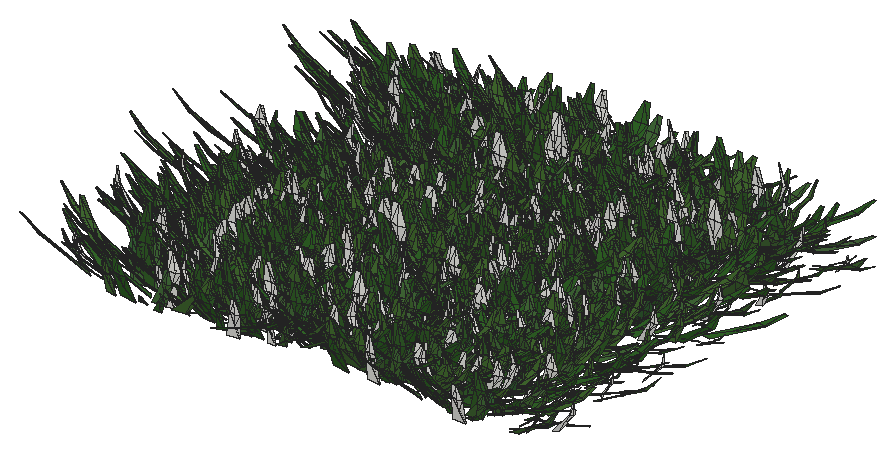
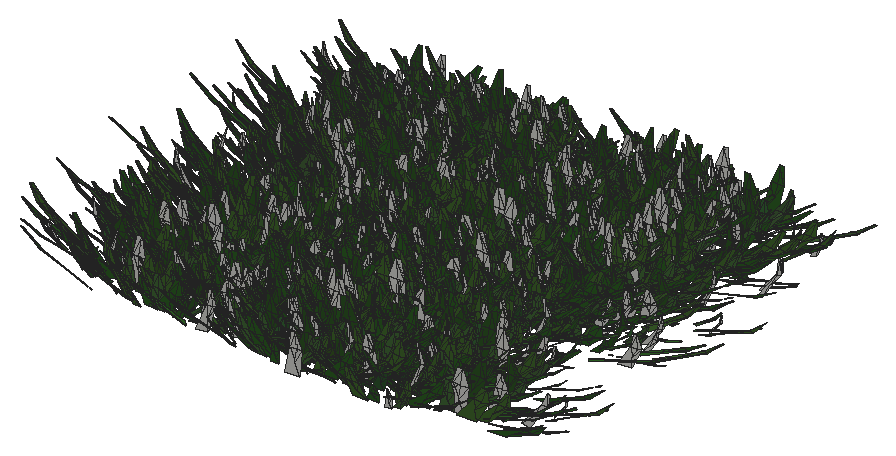
# SketchUp Ruby script. Lengths in inches.
U = 1.inch
M = Sketchup.active_model
def pt(a) = Geom::Point3d.new(a.map { |v| v * U })
def face(e, loops, mat)
  f = e.add_face(loops[0].map { |a| pt(a) })
  loops[1..].each { |l| e.add_face(l.map { |a| pt(a) }).erase! }
  f.material = f.back_material = mat if mat
  f
end
# faces: each face lists its corners as indices into pts; further lists are holes
def faces(e, pts, list, mat = nil) = list.each { |f| face(e, (f[0].is_a?(Array) ? f : [f]).map { |l| l.map { |i| pts[i] } }, mat) }
# xy, xz, yz: faces in a plane at the given z, y or x. An outline is a flat list of corners, or four numbers for a rectangle; further outlines are holes
def ring(l) = l.size == 4 ? [[l[0], l[1]], [l[2], l[1]], [l[2], l[3]], [l[0], l[3]]] : l.each_slice(2).to_a
def flat(e, list, mat, &to3) = list.each { |f| face(e, (f[0].is_a?(Array) ? f : [f]).map { |l| ring(l).map { |u, v| to3.(u, v) } }, mat) }
def xy(e, z, list, mat = nil) = flat(e, list, mat) { |x, y| [x, y, z] }
def xz(e, y, list, mat = nil) = flat(e, list, mat) { |x, z| [x, y, z] }
def yz(e, x, list, mat = nil) = flat(e, list, mat) { |y, z| [x, y, z] }
def lines(e, pts, list) = list.each { |a, b| e.add_line(pt(pts[a]), pt(pts[b])) }
# prism: a flat outline (further loops are holes) pulled along v
def prism(e, loops, v, mat = nil)
  f = face(e, loops, mat); d = Geom::Vector3d.new(v.map { |x| x * U })
  f.pushpull(f.normal.samedirection?(d) ? d.length : -d.length)
end
def box(e, o, s, mat = nil) = prism(e, [[o, [o[0] + s[0], o[1], o[2]], [o[0] + s[0], o[1] + s[1], o[2]], [o[0], o[1] + s[1], o[2]]]], [0, 0, s[2]], mat)
def at(x, y, z, deg = 0) = Geom::Transformation.translation(pt([x, y, z])) * Geom::Transformation.rotation(ORIGIN, Z_AXIS, deg.degrees)
def axes(o, x, y, z) = Geom::Transformation.new([*x, 0, *y, 0, *z, 0, *pt(o).to_a, 1])
def part(name) = M.definitions.add(name)
# library, detail: a bought-in or finely detailed component or shape, given as its bounding box
def library(name, o, s) = part(name).tap { |d| box(d.entities, o, s) }
def detail(e, o, s) = box(e.add_group.entities, o, s)
def put(e, d, t, mat = nil) = e.add_instance(d, t).tap { |i| i.material = mat if mat }
def group(e, t, mat = nil) = e.add_group.tap { |g| g.transformation = t; g.material = mat if mat }.entities
root = M.entities
M.materials.add("Material10").color = [48, 100, 38]
M.materials.add("Material3").color = [68, 110, 58]
M.materials.add("Material4").color = [48, 90, 38]
M.materials.add("Material5").color = [68, 110, 48]
M.materials.add("Material6").color = [48, 90, 48]
M.materials.add("Material7").color = [58, 110, 58]
M.materials.add("Material8").color = [58, 90, 38]
M.materials.add("Material9").color = [68, 100, 58]
c1 = part("grass00")
p = [[-0.6875,0.15,0],[-0.56,0.08,5.52],[-0.04,0.03,2.76],[0.48,-0.02,0],[0.35,-0.02,5.52],[-0.1,-0.14,5.52],
  [-0.12,0.65,8.37],[-0.42,0.65,8.37]]
faces(c1.entities,p,[[0,1,2,3],[3,2,4],[1,5,2],[5,4,2],[1,6,5],[4,5,6],[7,6,1]])
c2 = part("Group16\#1")
put(c2.entities,c1,axes([1.44,-0.61,-0.01],[0.05352,0.12609,0],[-0.10704,0.04543,0.07239],[0.06664,-0.02828,0.11628]),"Material6")
put(c2.entities,c1,axes([0.76,-0.15,-0.01],[0.04676,0.24062,0],[-0.23162,0.04501,0.06642],[0.0652,-0.01267,0.23595]),"Material3")
put(c2.entities,c1,axes([0.79,0.01,-0.01],[-0.00606,0.34651,0],[-0.34381,-0.00602,0.0432],[0.04319,0.00076,0.34386]))
put(c2.entities,c1,axes([1,0.23,-0.01],[-0.07192,0.31144,0],[-0.28722,-0.06632,0.1236],[0.12043,0.02781,0.29478]),"Material5")
put(c2.entities,c1,axes([1.66,0.77,-0.01],[-0.13828,0.29651,0],[-0.21551,-0.1005,0.22471],[0.20365,0.09498,0.23779]),"Material10")
put(c2.entities,c1,axes([0.6875,0.52,-0.01],[-0.18126,0.24051,0],[-0.22746,-0.17142,0.09788],[0.07817,0.05891,0.28481]),"Material5")
put(c2.entities,c1,axes([0.68,0.78,-0.01],[-0.215,0.18688,0],[-0.12385,-0.14248,0.21334],[0.13995,0.16101,0.18878]),"Material3")
put(c2.entities,c1,axes([0.56,1,-0.01],[-0.13756,0.07624,0],[-0.06159,-0.11112,0.0927],[0.04494,0.08108,0.12705]),"Material5")
put(c2.entities,c1,axes([0.2,0.64,-0.01],[-0.23729,0.07254,0],[-0.05711,-0.18681,0.153],[0.04473,0.14632,0.19535]),"Material10")
put(c2.entities,c1,axes([0.0625,0.72,-0.01],[-0.28874,0.02525,0],[-0.02179,-0.24916,0.14647],[0.01276,0.14591,0.25012]),"Material3")
put(c2.entities,c1,axes([-0.08,0.62,-0.01],[-0.34089,-0.04187,0],[0.03255,-0.26504,0.216],[-0.02633,0.21439,0.26703]),"Material10")
put(c2.entities,c1,axes([-0.34,0.98,-0.01],[-0.14314,-0.0493,0],[0.04397,-0.12769,0.06843],[-0.02228,0.0647,0.13505]),"Material10")
put(c2.entities,c1,axes([-0.87,1.45,-0.01],[-0.23488,-0.14114,0],[0.13761,-0.22901,0.06087],[-0.03135,0.05217,0.26717]))
put(c2.entities,c1,axes([-0.72,0.77,-0.01],[-0.14208,-0.13251,0],[0.07209,-0.0773,0.16301],[-0.11118,0.11922,0.1057]),"Material10")
put(c2.entities,c1,axes([-0.62,0.43,-0.01],[-0.14845,-0.21203,0],[0.18654,-0.13061,0.12304],[-0.10079,0.07057,0.22772]),"Material3")
put(c2.entities,c1,axes([-0.68,0.29,-0.01],[-0.13639,-0.32136,0],[0.31723,-0.13464,0.05579],[-0.05136,0.0218,0.34462]),"Material4")
put(c2.entities,c1,axes([-0.64,0.125,-0.01],[-0.0458,-0.23569,0],[0.22124,-0.043,0.08276],[-0.08124,0.01579,0.22538]),"Material7")
put(c2.entities,c1,axes([-1.6,-0.03,-0.01],[0.00576,-0.32897,0],[0.27526,0.00482,0.18018],[-0.18015,-0.00315,0.2753]),"Material5")
put(c2.entities,c1,axes([-1.36,-0.31,-0.01],[0.05718,-0.24765,0],[0.18172,0.04196,0.17267],[-0.16825,-0.03885,0.1865]),"Material10")
put(c2.entities,c1,axes([-1.54,-0.72,-0.01],[0.06537,-0.14017,0],[0.13555,0.06321,0.03939],[-0.0357,-0.01665,0.14956]))
put(c2.entities,c1,axes([-1.19,-0.9,-0.01],[0.09597,-0.12735,0],[0.11214,0.08451,0.07557],[-0.06035,-0.04548,0.14042]),"Material9")
put(c2.entities,c1,axes([-0.47,-0.54,-0.01],[0.11588,-0.10072,0],[0.0618,0.0711,0.12124],[-0.07953,-0.0915,0.0942]))
put(c2.entities,c1,axes([-0.47,-0.84,-0.01],[0.11927,-0.0661,0],[0.06603,0.11913,0.00646],[-0.00313,-0.00565,0.13621]),"Material5")
put(c2.entities,c1,axes([-0.38,-1.24,-0.01],[0.28037,-0.08571,0],[0.0618,0.20215,0.20315],[-0.05939,-0.19428,0.21139]),"Material9")
put(c2.entities,c1,axes([-0.06,-0.66,-0.01],[0.22719,-0.01987,0],[0.01247,0.14255,0.17758],[-0.01547,-0.17691,0.1431]),"Material8")
put(c2.entities,c1,axes([0.11,-0.89,-0.01],[0.14882,0.01828,0],[-0.01058,0.08611,0.12229],[0.01491,-0.12138,0.08676]),"Material6")
put(c2.entities,c1,axes([0.25,-0.72,-0.01],[0.20481,0.07053,0],[-0.06206,0.18022,0.10291],[0.03351,-0.0973,0.1906]),"Material6")
put(c2.entities,c1,axes([0.85,-1.42,-0.01],[0.16481,0.09904,0],[-0.09472,0.15762,0.05616],[0.02893,-0.04814,0.18389]),"Material5")
put(c2.entities,c1,axes([1.01,-1.09,-0.01],[0.21858,0.20385,0],[-0.17495,0.1876,0.15339],[0.10462,-0.11218,0.25652]),"Material10")
put(c2.entities,c1,axes([1.01,-0.71,-0.01],[0.08733,0.12473,0],[-0.06445,0.04512,0.13037],[0.1068,-0.07477,0.07867]),"Material6")
c3 = part("Group15\#1")
put(c3.entities,c2,at(0,0,0))
c4 = part("3darcstudiotree_grass00\#1")
put(c4.entities,c3,at(0,0,0))
put(root,c4,axes([226.21,4.08,7.6],[3.20529,-0.95815,0],[3.41522,0.71406,-0.02296],[0.11616,0.02429,1.8355]))
put(root,c4,axes([225.98,41.5625,7.6],[-1.06603,0.92748,0],[-4.93521,-0.35453,-0.06106],[-0.26936,-0.01935,1.47293]))
put(root,c4,axes([225.79,20.19,7.6],[5.08676,-0.19422,0],[0.58185,0.95246,-0.02943],[0.02798,0.0458,1.51666]))
put(root,c4,axes([227.38,18.53,7.6],[-0.19939,-1.04542,0],[4.4829,-0.05344,-0.05646],[0.31576,-0.00376,1.57058]))
put(root,c4,axes([225.93,11.33,7.6],[2.71383,0.81638,0],[-3.43896,0.71449,-0.05468],[-0.2392,0.0497,1.58958]))
put(root,c4,axes([225.9,26.8,7.6],[4.84098,0.43489,0],[-1.61189,1.12141,-0.03831],[-0.06664,0.04636,1.53223]))
put(root,c4,axes([226.47,38.5,7.6],[4.94595,-0.11829,0],[0.37031,0.96768,-0.00501],[0.00319,0.00833,1.62495]))
put(root,c4,axes([226.14,12.84,7.6],[2.55592,1.10469,0],[-4.04438,0.58485,-0.02506],[-0.13578,0.01964,1.82822]))
put(root,c4,axes([226.78,7.125,7.6],[4.08301,-0.07651,0],[0.38191,1.27383,-0.00347],[0.00157,0.00523,1.92949]))
put(root,c4,axes([227.87,35.8,7.6],[-2.35704,0.79519,0],[-3.72282,-0.68968,-0.05517],[-0.2648,-0.04906,1.72999]))
put(root,c4,axes([227.11,17.55,7.6],[2.61917,0.95948,0],[-3.03892,0.51848,-0.01403],[-0.09978,0.01702,1.97952]))
put(root,c4,axes([227.21,23.57,7.6],[3.34714,0.66833,0],[-2.79001,0.87331,-0.04015],[-0.12528,0.03922,1.39698]))
put(root,c4,axes([227.82,14.5625,7.6],[0.48467,1.00987,0],[-3.72895,0.11185,-0.01784],[-0.13598,0.00408,1.80168]))
put(root,c4,axes([229.61,33.6875,7.6],[-1.59666,-0.99905,0],[3.40836,-0.34045,-0.01431],[0.10062,-0.01005,1.73701]))
put(root,c4,axes([229.78,5.64,7.6],[-3.03643,0.87412,0],[-2.8621,-0.62138,-0.01448],[-0.06458,-0.01402,1.39954]))
put(root,c4,axes([230.84,6.7,7.6],[-4.02149,-0.43578,0],[1.45299,-0.83803,-0.04544],[0.11799,-0.06805,1.4908]))
put(root,c4,axes([231.12,29.33,7.6],[-4.89707,0.28407,0],[-0.88262,-0.95096,-0.03599],[-0.04789,-0.0516,1.43677]))
put(root,c4,axes([230.44,14.26,7.6],[-3.37258,0.90608,0],[-3.64602,-0.8482,-0.01383],[-0.04832,-0.01124,1.48532]))
put(root,c4,axes([229.94,22.19,7.6],[4.28972,0.40809,0],[-1.53876,1.01093,-0.01203],[-0.02546,0.01673,1.60927]))
put(root,c4,axes([231.98,18.82,7.6],[-1.14965,-0.87516,0],[3.85465,-0.31648,-0.02104],[0.11481,-0.00943,1.45661]))
put(root,c4,axes([231.18,16.43,7.6],[3.45148,-0.64536,0],[2.96079,0.98967,-0.02614],[0.07518,0.02513,1.48366]))
put(root,c4,axes([232.02,20.76,7.6],[-4.9983,0.12378,0],[-0.36429,-0.91937,-0.0174],[-0.01281,-0.03234,1.72585]))
put(root,c4,axes([232.56,38.6,7.6],[-3.38152,-0.37053,0],[1.95757,-1.11657,-0.00176],[0.00453,-0.00258,1.95594]))
put(root,c4,axes([231.52,11.12,7.6],[-2.34957,0.94392,0],[-4.17021,-0.64877,-0.04897],[-0.26523,-0.04126,1.9584]))
put(root,c4,axes([230.93,8.84,7.6],[3.32402,0.3596,0],[-1.44399,0.83424,-0.02703],[-0.09074,0.05242,1.9211]))
put(root,c4,axes([232.95,26.33,7.6],[-3.05623,-0.47682,0],[2.41216,-0.96631,-0.00523],[0.01811,-0.00725,1.86317]))
put(root,c4,axes([233.09,28.7,7.6],[-3.75382,-0.50938,0],[2.09214,-0.9636,-0.04387],[0.13012,-0.05993,1.70431]))
put(root,c4,axes([232.33,9.76,7.6],[-3.73599,0.53776,0],[-2.5701,-1.11595,-0.0199],[-0.05158,-0.02239,1.67187]))
put(root,c4,axes([231.25,25.49,7.6],[1.67846,0.81167,0],[-4.27264,0.55222,-0.03477],[-0.1745,0.02255,1.69826]))
put(root,c4,axes([232.66,17.13,7.6],[-3.09646,0.77516,0],[-3.18498,-0.79517,-0.05526],[-0.23608,-0.05894,1.69871]))
put(root,c4,axes([232.67,12.55,7.6],[2.62671,-0.96021,0],[3.1714,0.54222,-0.02882],[0.14083,0.02408,1.42183]))
put(root,c4,axes([233.14,43.38,7.6],[0.41254,-1.11538,0],[3.92373,0.0907,-0.04487],[0.25663,0.00593,1.41449]))
put(root,c4,axes([233.58,42.34,7.6],[-4.83141,-0.06367,0],[0.25709,-1.21932,-0.0488],[0.01394,-0.06614,1.65721]))
put(root,c4,axes([233.43,4.38,7.6],[-3.80323,0.13534,0],[-0.55678,-0.97788,-0.03826],[-0.03613,-0.06345,1.65468]))
put(root,c4,axes([234.05,39.82,7.6],[-4.67907,-0.20575,0],[0.86048,-1.22305,-0.04722],[0.03699,-0.05257,1.40384]))
put(root,c4,axes([232.57,36.71,7.6],[-1.05875,1.15742,0],[-4.29725,-0.24568,-0.0233],[-0.13048,-0.00746,1.58282]))
put(root,c4,axes([232.625,23.74,7.6],[4.14871,0.66652,0],[-2.80307,1.09047,-0.03131],[-0.07779,0.03026,1.48921]))
put(root,c4,axes([232.9,32.76,7.6],[2.97201,1.00736,0],[-3.97981,0.73385,-0.05484],[-0.18767,0.03461,1.31443]))
put(root,c4,axes([233.51,31.37,7.6],[3.73635,0.02915,0],[-0.121,0.9694,-0.01718],[-0.00416,0.0333,1.88076]))
put(root,c4,axes([235.78,16.42,7.6],[-3.38708,-0.63927,0],[2.81669,-0.93274,-0.01411],[0.04933,-0.01634,1.69584]))
put(root,c4,axes([233.76,35.375,7.6],[0.16986,1.07544,0],[-5.18803,0.05121,-0.04149],[-0.19714,0.00195,1.54325]))
put(root,c4,axes([235.98,29.46,7.6],[0.73918,-1.25402,0],[4.5803,0.16874,-0.00777],[0.03593,0.00132,1.3523]))
put(root,c4,axes([236.16,26.67,7.6],[-0.83171,-0.90909,0],[4.59832,-0.26293,-0.04627],[0.28513,-0.0163,1.86363]))
put(root,c4,axes([236.2,17.17,7.6],[-4.52783,0.09424,0],[-0.31079,-0.93327,-0.02559],[-0.01771,-0.05318,1.95328]))
put(root,c4,axes([237.05,25.02,7.6],[1.09611,-0.92163,0],[4.84666,0.36027,-0.06029],[0.32691,0.0243,1.78762]))
put(root,c4,axes([236.72,39.72,7.6],[2.30561,-0.85947,0],[4.07199,0.68272,-0.05795],[0.30529,0.05118,1.94389]))
put(root,c4,axes([236.01,8.4,7.6],[4.15645,0.11327,0],[-0.40548,0.92998,-0.03498],[-0.02406,0.05518,1.48455]))
put(root,c4,axes([236.93,21.94,7.6],[-3.28835,0.69112,0],[-2.3207,-0.69011,-0.00081],[-0.00409,-0.00122,1.76997]))
put(root,c4,axes([238.16,34.58,7.6],[-0.05217,-0.99103,0],[4.9332,-0.01623,-0.00745],[0.04692,-0.00015,1.94284]))
put(root,c4,axes([236.73,5.44,7.6],[0.29849,1.1081,0],[-3.91006,0.06583,-0.04154],[-0.31526,0.00531,1.86323]))
put(root,c4,axes([238.3125,31.26,7.6],[-4.94093,-0.24625,0],[0.95755,-1.20083,-0.01918],[0.02332,-0.02924,1.90358]))
put(root,c4,axes([236.96,36.09,7.6],[3.27459,-0.53526,0],[2.01,0.76855,-0.045],[0.14728,0.05631,1.37282]))
put(root,c4,axes([238.37,20.79,7.6],[0.57888,-1.02767,0],[4.86352,0.17122,-0.00524],[0.03332,0.00117,1.97007]))
put(root,c4,axes([236.5,13.46,7.6],[1.77436,0.79751,0],[-3.18659,0.44311,-0.00131],[-0.00977,0.00136,1.9458]))
put(root,c4,axes([237.62,6.83,7.6],[-3.36301,0.64766,0],[-2.44825,-0.79454,-0.00087],[-0.00355,-0.00115,1.68429]))
put(root,c4,axes([238.76,11.24,7.6],[-1.4545,-0.88118,0],[4.51048,-0.46532,-0.01762],[0.07914,-0.00816,1.48208]))
put(root,c4,axes([236.68,9.58,7.6],[3.81768,0.66428,0],[-2.44879,0.87959,-0.01513],[-0.0462,0.0166,1.43215]))
put(root,c4,axes([237.86,32.56,7.6],[4.08726,-0.46656,0],[1.95644,1.0712,-0.05401],[0.10986,0.06015,1.44188]))
put(root,c4,axes([239.67,41.65,7.6],[-3.9964,-0.52288,0],[2.12612,-1.01563,-0.05348],[0.15903,-0.07597,1.83786]))
put(root,c4,axes([238.24,23.72,7.6],[4.81145,-0.0979,0],[0.38638,1.1868,-0.02372],[0.00959,0.02946,1.48337]))
put(root,c4,axes([239.875,42.75,7.6],[-4.62401,0.29061,0],[-0.94259,-0.93738,-0.03206],[-0.05298,-0.05269,1.63785]))
put(root,c4,axes([238.8,37.05,7.6],[2.68838,0.69195,0],[-3.43987,0.83529,-0.03466],[-0.15751,0.03825,1.89896]))
put(root,c4,axes([238.85,27.94,7.6],[3.81617,0.61886,0],[-2.68846,1.03615,-0.05832],[-0.15316,0.05903,1.48992]))
put(root,c4,axes([239.43,38.9,7.6],[-0.04272,0.99569,0],[-4.10213,-0.011,-0.03184],[-0.21296,-0.00057,1.71482]))
put(root,c4,axes([239.85,19.24,7.6],[-2.13592,1.02189,0],[-4.55643,-0.59523,-0.06253],[-0.32722,-0.04275,1.89715]))
put(root,c4,axes([239.74,14.65,7.6],[3.87992,-0.06992,0],[0.26674,0.92505,-0.00836],[0.00512,0.01775,1.97523]))
put(root,c4,axes([242.15,26.7,7.6],[-3.92726,-0.53289,0],[2.331,-1.07368,-0.04044],[0.11775,-0.05424,1.86421]))
put(root,c4,axes([242.45,23.54,7.6],[-4.06696,-0.33259,0],[1.16201,-0.88807,-0.035],[0.08068,-0.06166,1.73222]))
put(root,c4,axes([243.06,37.53,7.6],[-4.12513,-0.57559,0],[2.48785,-1.11437,-0.0179],[0.04452,-0.01994,1.62858]))
put(root,c4,axes([242.14,11.38,7.6],[-3.59802,0.5872,0],[-2.6694,-1.02229,-0.04574],[-0.15156,-0.05804,1.85022]))
put(root,c4,axes([242.96,10.45,7.6],[0.47235,-1.15777,0],[4.32597,0.11031,-0.00761],[0.05408,0.00138,1.94156]))
put(root,c4,axes([243.24,29.25,7.6],[-3.32765,-0.85792,0],[3.0305,-0.73466,-0.04714],[0.2036,-0.04936,1.58733]))
put(root,c4,axes([241.69,7.93,7.6],[5.16492,-0.13655,0],[0.53557,1.26611,-0.02611],[0.01692,0.04001,1.96192]))
put(root,c4,axes([242.89,31.01,7.6],[-3.3634,0.85391,0],[-3.17768,-0.78227,-0.02428],[-0.08249,-0.02031,1.32917]))
put(root,c4,axes([243.89,13.48,7.6],[-3.44,-0.36745,0],[1.97613,-1.15625,-0.04539],[0.10919,-0.06389,1.92461]))
put(root,c4,axes([242.49,43.7,7.6],[4.78852,-0.11236,0],[0.42706,1.13749,-0.03728],[0.02321,0.06182,1.90298]))
put(root,c4,axes([242.87,39.84,7.6],[4.63211,-0.48455,0],[1.59506,0.95302,-0.04818],[0.10631,0.06352,1.47658]))
put(root,c4,axes([243.15,39.17,7.6],[3.86267,-0.07613,0],[0.40494,1.28409,-0.03935],[0.01388,0.04402,1.44542]))
put(root,c4,axes([243.95,33.81,7.6],[2.43686,-0.68298,0],[3.57771,0.79783,-0.04874],[0.17486,0.03899,1.44038]))
put(root,c4,axes([243.08,16.0625,7.6],[4.82681,-0.00126,0],[0.00513,1.22505,-0.04894],[0.00024,0.05639,1.41164]))
put(root,c4,axes([245.16,28.69,7.6],[-3.42276,-0.65167,0],[2.58269,-0.84782,-0.01582],[0.04944,-0.01623,1.37394]))
put(root,c4,axes([244.01,25.6,7.6],[-2.36541,1.04526,0],[-3.84689,-0.54409,-0.02589],[-0.11432,-0.01617,1.40149]))
put(root,c4,axes([244.54,41.82,7.6],[2.7424,-0.7825,0],[2.89337,0.63377,-0.00209],[0.01007,0.00221,1.54397]))
put(root,c4,axes([244.71,36.02,7.6],[-4.1603,0.72793,0],[-2.33598,-0.83442,-0.01309],[-0.05536,-0.01977,1.87779]))
put(root,c4,axes([245.44,15.04,7.6],[-0.84808,-1.10481,0],[3.74786,-0.17981,-0.00431],[0.02392,-0.00115,1.34772]))
put(root,c4,axes([245.75,5.84,7.6],[-1.71072,-0.80836,0],[3.80701,-0.50355,-0.0302],[0.16613,-0.02197,1.67548]))
put(root,c4,axes([245.84,18.85,7.6],[0.18531,-0.97415,0],[3.90679,0.04645,-0.0123],[0.08869,0.00105,1.7643]))
put(root,c4,axes([244.55,21.84,7.6],[3.52409,0.23962,0],[-1.16841,1.07399,-0.02379],[-0.03363,0.03091,1.49895]))
put(root,c4,axes([244.29,17.48,7.6],[1.29524,0.85298,0],[-4.77119,0.45281,-0.02635],[-0.13125,0.01246,1.69955]))
put(root,c4,axes([246.11,32.66,7.6],[-4.98991,0.20865,0],[-0.7989,-1.19409,-0.00717],[-0.00589,-0.0088,1.50735]))
put(root,c4,axes([245.55,20.92,7.6],[2.92176,-0.52894,0],[2.46205,0.84999,-0.04376],[0.17079,0.05896,1.7457]))
put(root,c4,axes([247.85,26.18,7.6],[-2.67053,-0.99485,0],[3.36476,-0.56452,-0.00883],[0.05512,-0.00925,1.90461]))
put(root,c4,axes([248.26,38.97,7.6],[-2.95255,-0.81537,0],[3.60487,-0.81585,-0.01753],[0.06331,-0.01433,1.48083]))
put(root,c4,axes([246.02,6.95,7.6],[-0.18508,1.23432,0],[-4.73712,-0.04439,-0.00219],[-0.0103,-0.0001,1.39308]))
put(root,c4,axes([248.47,9.48,7.6],[-4.20317,-0.73758,0],[2.25744,-0.80401,-0.02484],[0.09654,-0.03438,1.66133]))
put(root,c4,axes([248.13,34.7,7.6],[-4.46812,0.07741,0],[-0.25002,-0.9019,-0.01842],[-0.00759,-0.0274,1.34789]))
put(root,c4,axes([248.66,5.71,7.6],[-3.42874,0.45159,0],[-1.78492,-0.84701,-0.01732],[-0.06439,-0.03056,1.90951]))
put(root,c4,axes([249.98,42.04,7.6],[-1.47134,-1.07173,0],[4.62951,-0.39723,-0.00214],[0.01137,-0.00098,1.72072]))
put(root,c4,axes([247.86,10.95,7.6],[4.20048,0.55778,0],[-1.88075,0.88521,-0.04207],[-0.14917,0.07021,1.89419]))
put(root,c4,axes([248.32,22.125,7.6],[2.35176,0.86373,0],[-3.11236,0.52965,-0.02533],[-0.14132,0.02405,1.58831]))
put(root,c4,axes([248.98,37.62,7.6],[4.3887,-0.53019,0],[1.93978,1.00355,-0.00312],[0.00847,0.00438,1.73901]))
put(root,c4,axes([248.65,17.62,7.6],[1.01063,1.23996,0],[-4.41491,0.2249,-0.0503],[-0.27557,0.01404,1.57458]))
put(root,c4,axes([249.02,28.07,7.6],[-1.65132,1.02753,0],[-4.1479,-0.41662,-0.02547],[-0.11726,-0.01178,1.38631]))
put(root,c4,axes([250.17,15.56,7.6],[0.96836,-1.19447,0],[4.79826,0.24312,-0.041],[0.23189,0.01175,1.76588]))
put(root,c4,axes([248.88,12.71,7.6],[4.53801,0.33747,0],[-1.32832,1.11639,-0.03162],[-0.04162,0.03498,1.3441]))
put(root,c4,axes([248.72,23.21,7.6],[2.33175,0.74132,0],[-3.89169,0.76506,-0.01217],[-0.05632,0.01107,1.82194]))
put(root,c4,axes([250.44,6.48,7.6],[1.73115,-0.99463,0],[4.00302,0.43545,-0.04597],[0.21468,0.02335,1.38947]))
put(root,c4,axes([251.42,8.78,7.6],[-4.68105,-0.44507,0],[1.39415,-0.91644,-0.04106],[0.1024,-0.06731,1.71966]))
put(root,c4,axes([251.33,39.96,7.6],[-4.10991,0.05659,0],[-0.25803,-1.17127,-0.02509],[-0.00633,-0.02875,1.34616]))
put(root,c4,axes([252.04,33.26,7.6],[-0.81845,-1.22057,0],[4.38476,-0.18376,-0.02808],[0.16711,-0.007,1.67665]))
put(root,c4,axes([251.22,20.23,7.6],[2.60124,-1.09423,0],[3.31981,0.49325,-0.0411],[0.22316,0.03316,1.52451]))
put(root,c4,axes([250.34,29.58,7.6],[3.5289,0.32153,0],[-1.76569,1.21119,-0.03532],[-0.06738,0.04622,1.79519]))
put(root,c4,axes([250.87,25.67,7.6],[0.58187,0.98724,0],[-3.75225,0.13822,-0.04131],[-0.23221,0.00855,1.34689]))
put(root,c4,axes([251.41,19.57,7.6],[4.31659,-0.72181,0],[2.02591,0.75722,-0.03191],[0.13976,0.05224,1.79443]))
put(root,c4,axes([251.83,14.52,7.6],[3.90895,-0.31621,0],[1.44431,1.11591,-0.01717],[0.02682,0.02072,1.48777]))
put(root,c4,axes([251.91,30.76,7.6],[0.60806,1.1895,0],[-3.81317,0.12183,-0.04145],[-0.33743,0.01078,1.97198]))
put(root,c4,axes([251.64,35.61,7.6],[4.01339,0.62208,0],[-2.19682,0.88582,-0.03504],[-0.13521,0.05452,1.90819]))
put(root,c4,axes([254.07,9.89,7.6],[-1.20844,-0.99932,0],[4.83991,-0.36579,-0.03772],[0.15637,-0.01182,1.36861]))
put(root,c4,axes([253.84,30.65,7.6],[-2.41677,0.79192,0],[-3.38406,-0.64546,-0.05103],[-0.26235,-0.05004,1.72023]))
put(root,c4,axes([254.35,39,7.6],[-3.63977,0.77847,0],[-2.95769,-0.8643,-0.05065],[-0.16741,-0.04892,1.44592]))
put(root,c4,axes([255.54,28.41,7.6],[-3.02666,-0.90444,0],[3.4297,-0.71733,-0.01878],[0.08665,-0.01812,1.68146]))
put(root,c4,axes([255.78,23.36,7.6],[-3.4696,-0.46787,0],[1.78358,-0.82666,-0.04409],[0.13229,-0.06131,1.48398]))
put(root,c4,axes([255.52,29.15,7.6],[-4.56638,0.55078,0],[-1.82444,-0.94538,-0.02532],[-0.06885,-0.03568,1.64221]))
put(root,c4,axes([254.38,43.25,7.6],[4.17819,0.33382,0],[-1.2451,0.97401,-0.03842],[-0.08739,0.06836,1.90991]))
put(root,c4,axes([255.05,18.54,7.6],[4.13559,-0.54308,0],[1.81906,0.86577,-0.02304],[0.07821,0.03723,1.78453]))
put(root,c4,axes([256.72,37.43,7.6],[0.6928,-1.22893,0],[4.48898,0.15816,-0.02402],[0.15455,0.00545,1.84088]))
put(root,c4,axes([256.88,12.625,7.6],[-4.87146,0.02178,0],[-0.08116,-1.13448,-0.01042],[-0.0012,-0.01672,1.82123]))
put(root,c4,axes([256.86,5.08,7.6],[-3.73268,0.3096,0],[-1.29853,-0.97848,-0.04681],[-0.08807,-0.06636,1.53984]))
put(root,c4,axes([255.5,11.77,7.6],[3.88196,0.27706,0],[-1.31813,1.15428,-0.00872],[-0.01209,0.01059,1.51538]))
put(root,c4,axes([256.1875,32.59,7.6],[-0.31756,1.20415,0],[-3.66526,-0.06041,-0.03816],[-0.32346,-0.00533,1.95014]))
put(root,c4,axes([255.33,8.16,7.6],[3.73866,0.84444,0],[-2.52225,0.69793,-0.00582],[-0.02595,0.00718,1.56404]))
put(root,c4,axes([255.47,16.1,7.6],[3.21656,0.87415,0],[-3.40413,0.78287,-0.033],[-0.15769,0.03627,1.87715]))
put(root,c4,axes([257.84,17.1875,7.6],[-1.25696,-0.97634,0],[4.48228,-0.36066,-0.0477],[0.21367,-0.01719,1.385]))
put(root,c4,axes([258.27,7.37,7.6],[-2.73694,-0.75436,0],[3.09304,-0.70138,-0.0539],[0.21901,-0.04966,1.43163]))
put(root,c4,axes([256.5,20.93,7.6],[3.21354,0.61237,0],[-2.33536,0.76595,-0.01463],[-0.06404,0.021,1.73802]))
put(root,c4,axes([256.63,15.03,7.6],[3.81718,0.38538,0],[-1.70529,1.05566,-0.03343],[-0.08298,0.05137,1.88641]))
put(root,c4,axes([257.14,41.78,7.6],[-0.16779,1.03236,0],[-3.91072,-0.03973,-0.03031],[-0.21719,-0.00221,1.75443]))
put(root,c4,axes([256.81,27.1,7.6],[3.62954,0.33152,0],[-1.65878,1.13506,-0.04863],[-0.08609,0.05891,1.5585]))
put(root,c4,axes([258.15,40.8,7.6],[-4.32193,0.57757,0],[-2.28366,-1.06804,-0.02635],[-0.05701,-0.02666,1.3895]))
put(root,c4,axes([256.64,35.61,7.6],[2.41826,1.00361,0],[-4.45314,0.67064,-0.01693],[-0.07141,0.01075,1.59984]))
put(root,c4,axes([257.45,24.71,7.6],[4.97151,0.37477,0],[-1.19031,0.98689,-0.04516],[-0.09125,0.07566,1.80387]))
put(root,c4,axes([258.22,33.6875,7.6],[-2.49241,1.02032,0],[-4.21954,-0.64421,-0.0342],[-0.15461,-0.0236,1.63693]))
